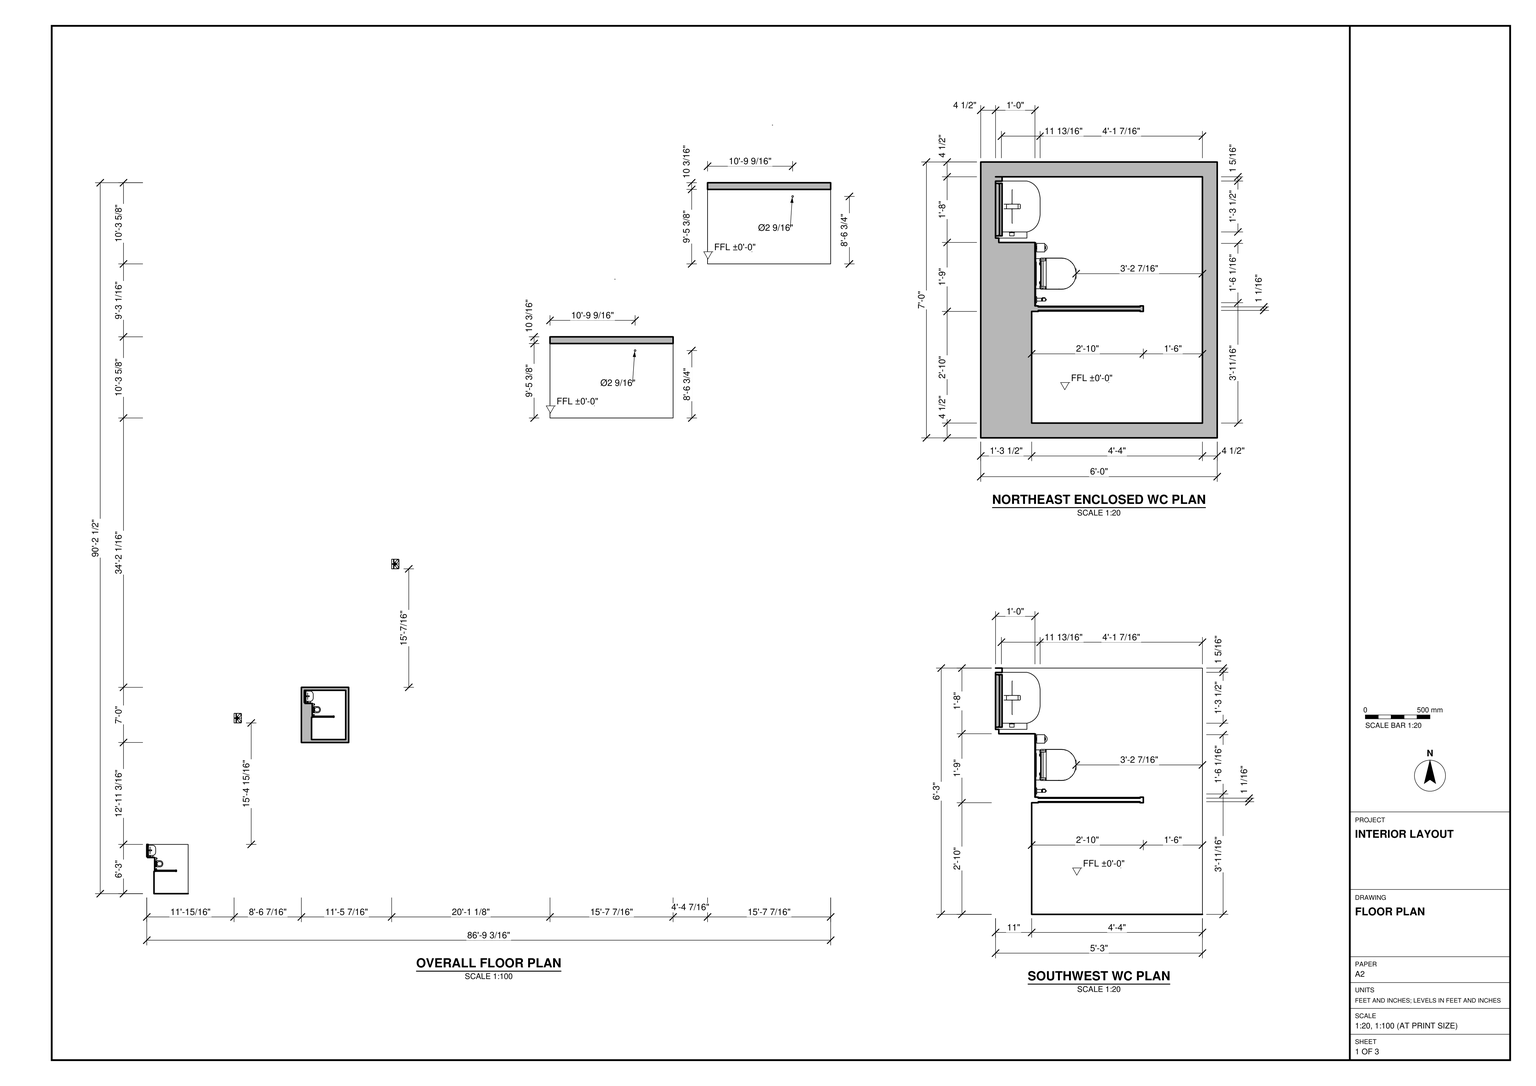
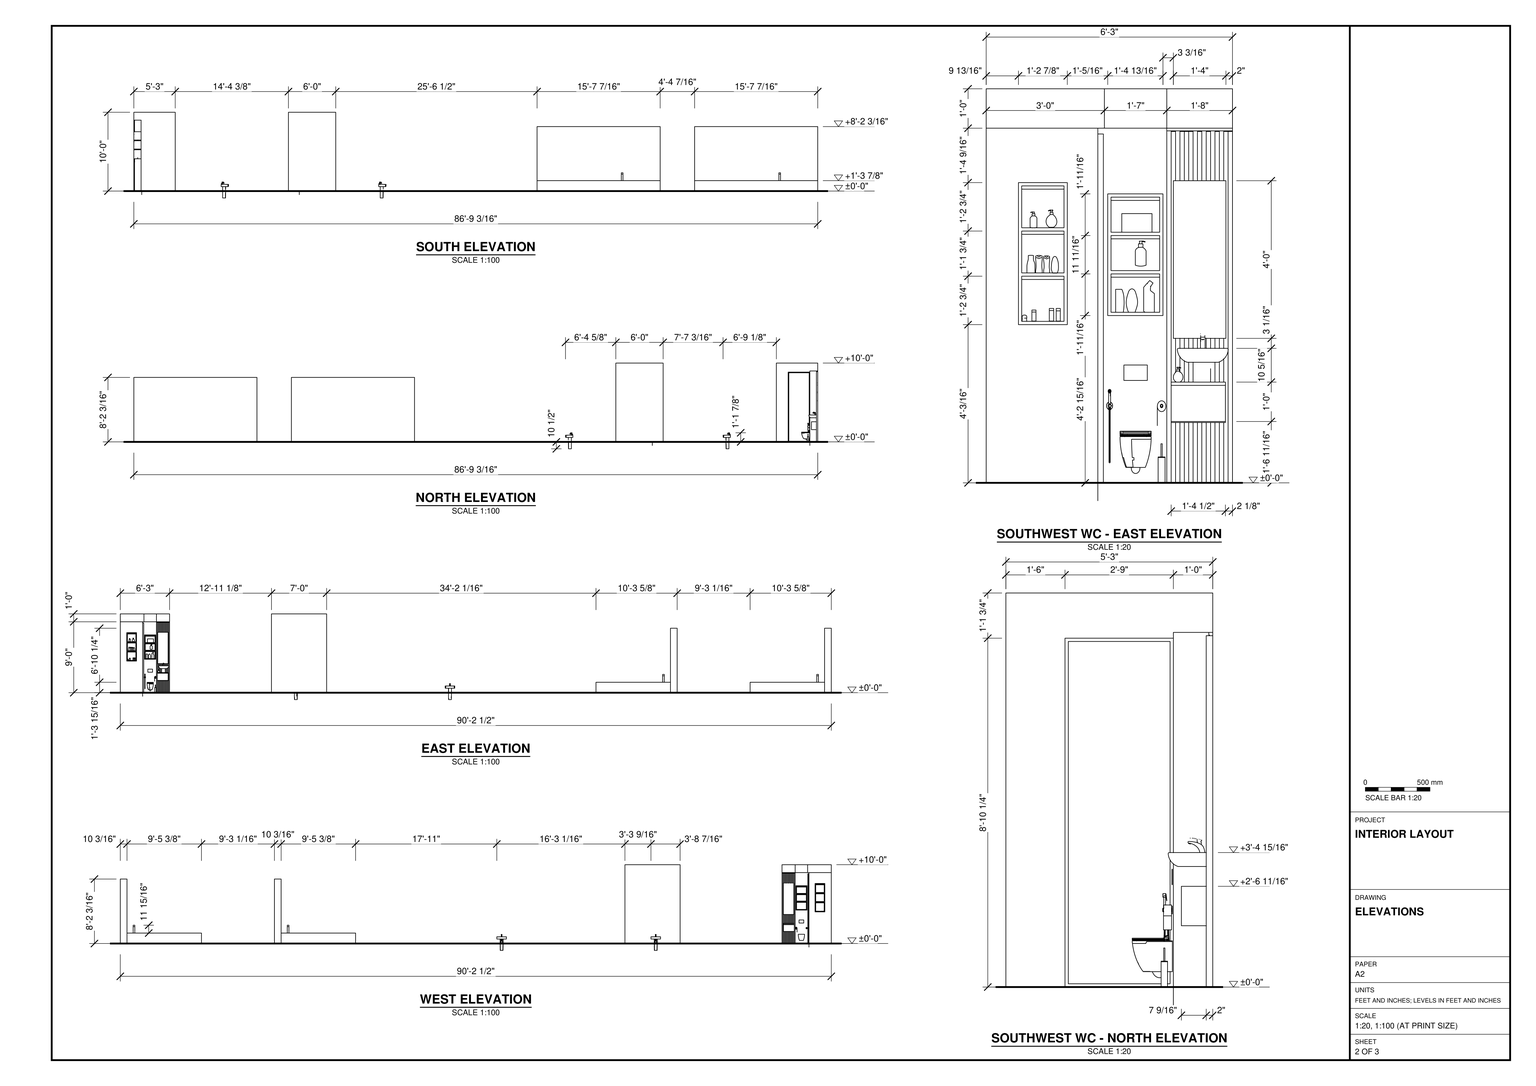
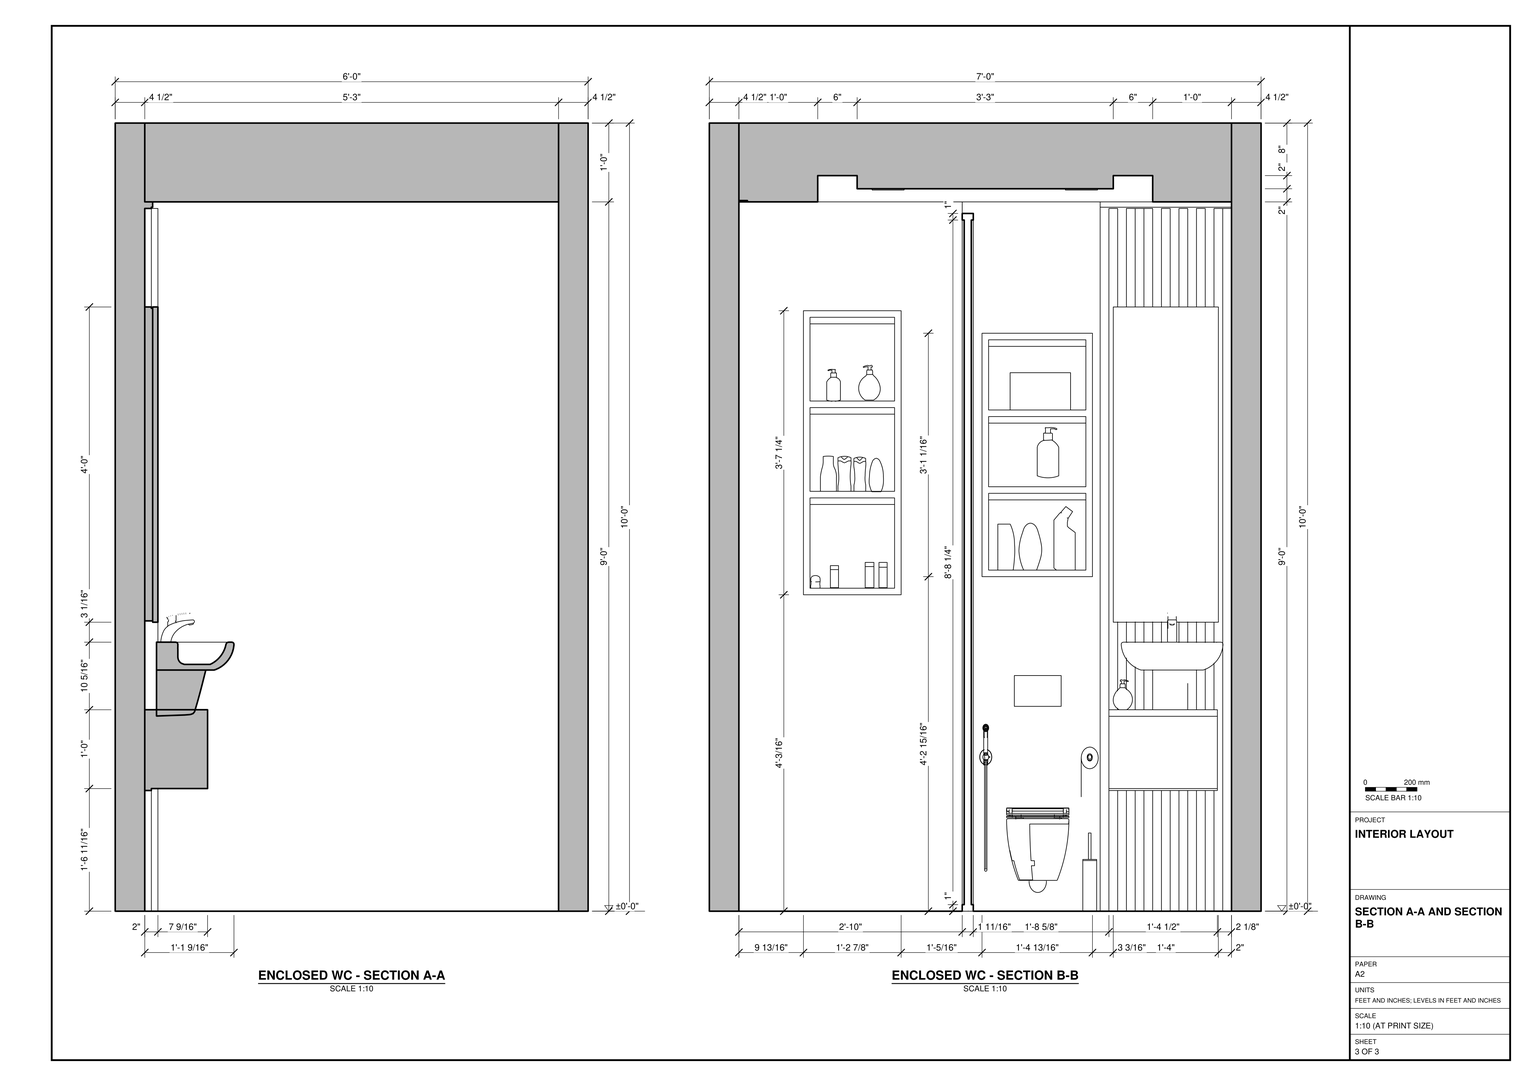
Build the interior layout in SketchUp from task_files/diagram_01.pdf. Work in feet and inches. Use the overall plan to position the separate assemblies; the spaces between them are part of the layout. The overall size is 86'-9 3/16" along x, 90'-2 1/2" along y and 10'-10 1/2" along z. Use the single finished floor level of ±0'-0".

Model the open southwest WC and the enclosed WC to its northeast. Use the enlarged plans for the stepped fixture wall and projecting partition. For the enclosed version, use the sections to set the perimeter wall thickness, ceiling height and stepped underside of the top slab. Fit both layouts with the wall-hung toilet, basin and tap, suspended cabinet, mirror, vertically lined backing and recessed shelves. Match the shelf sizes and the elevations of the basin fittings to the detail drawings. Decor and loose items, including containers on the shelves, may be any suitable library components.

Include the detached basin fixtures and the two larger rectangular assemblies farther northeast, each with a low base and a tall end panel. Keep the shell elements, including walls and slabs, and each furniture or joinery piece in separate groups or components. Use components for repeated parts. Save one SketchUp model as output_files/open_and_enclosed_wc_layouts_and_separate_fixtures.skp.

# SketchUp Ruby script. Lengths in inches.
U = 1.inch
M = Sketchup.active_model
def pt(a) = Geom::Point3d.new(a.map { |v| v * U })
def face(e, loops, mat)
  f = e.add_face(loops[0].map { |a| pt(a) })
  loops[1..].each { |l| e.add_face(l.map { |a| pt(a) }).erase! }
  f.material = f.back_material = mat if mat
  f
end
# faces: each face lists its corners as indices into pts; further lists are holes
def faces(e, pts, list, mat = nil) = list.each { |f| face(e, (f[0].is_a?(Array) ? f : [f]).map { |l| l.map { |i| pts[i] } }, mat) }
# xy, xz, yz: faces in a plane at the given z, y or x. An outline is a flat list of corners, or four numbers for a rectangle; further outlines are holes
def ring(l) = l.size == 4 ? [[l[0], l[1]], [l[2], l[1]], [l[2], l[3]], [l[0], l[3]]] : l.each_slice(2).to_a
def flat(e, list, mat, &to3) = list.each { |f| face(e, (f[0].is_a?(Array) ? f : [f]).map { |l| ring(l).map { |u, v| to3.(u, v) } }, mat) }
def xy(e, z, list, mat = nil) = flat(e, list, mat) { |x, y| [x, y, z] }
def xz(e, y, list, mat = nil) = flat(e, list, mat) { |x, z| [x, y, z] }
def yz(e, x, list, mat = nil) = flat(e, list, mat) { |y, z| [x, y, z] }
def lines(e, pts, list) = list.each { |a, b| e.add_line(pt(pts[a]), pt(pts[b])) }
# prism: a flat outline (further loops are holes) pulled along v
def prism(e, loops, v, mat = nil)
  f = face(e, loops, mat); d = Geom::Vector3d.new(v.map { |x| x * U })
  f.pushpull(f.normal.samedirection?(d) ? d.length : -d.length)
end
def box(e, o, s, mat = nil) = prism(e, [[o, [o[0] + s[0], o[1], o[2]], [o[0] + s[0], o[1] + s[1], o[2]], [o[0], o[1] + s[1], o[2]]]], [0, 0, s[2]], mat)
def at(x, y, z, deg = 0) = Geom::Transformation.translation(pt([x, y, z])) * Geom::Transformation.rotation(ORIGIN, Z_AXIS, deg.degrees)
def axes(o, x, y, z) = Geom::Transformation.new([*x, 0, *y, 0, *z, 0, *pt(o).to_a, 1])
def part(name) = M.definitions.add(name)
# library, detail: a bought-in or finely detailed component or shape, given as its bounding box
def library(name, o, s) = part(name).tap { |d| box(d.entities, o, s) }
def detail(e, o, s) = box(e.add_group.entities, o, s)
def put(e, d, t, mat = nil) = e.add_instance(d, t).tap { |i| i.material = mat if mat }
def group(e, t, mat = nil) = e.add_group.tap { |g| g.transformation = t; g.material = mat if mat }.entities
root = M.entities
M.materials.add("[0020_Red]").color = [255, 0, 0]
M.materials.add("[Carrera Marble]").color = [207, 207, 207]
M.materials.add("[Color M09]").color = [0, 0, 0]
M.materials.add("[Color_000]").color = [255, 234, 104]
M.materials.add("[Color_A02]").color = [255, 50, 50]
M.materials.add("[Color_B06]").color = [163, 8, 0]
M.materials.add("[Color_C10]").color = [125, 119, 117]
M.materials.add("[Color_I11]").color = [2, 32, 114]
M.materials.add("[Mirror 01]").color = [185, 185, 185]
M.materials.add("[Terrazzo Tile Accent]").color = [224, 221, 217]
M.materials.add("[Translucent Glass Sky Reflection]").color = [126, 138, 183]
M.materials["[Translucent Glass Sky Reflection]"].alpha = 0.52
M.materials.add("[Wood Veneer 01]").color = [120, 70, 37]
c1 = library("Wall-hung toilet assembly",[0,0,0],[28.35,19.69,42.125])
c2 = library("33.dxf",[36.1875,14.52,12],[23.625,39.43,18.1])
c3 = library("washbasin-1",[-10.81,-16.44,-15.75],[21.62,16.44,23.34])
c4 = library("Group\#4",[0,0,0],[5.59,14.85,1.64])
c5 = library("Group\#6",[0,0,0],[7.39,15.23,1.95])
c6 = library("Group\#10",[0,0,-0.06],[5.12,14.5,1.72])
c7 = library("Group\#7",[0,0,0],[9.4,15.15,3.11])
c8 = library("Group\#11",[0,0,0],[9.4,3.11,15.15])
c9 = library("Group\#12",[0,0,0],[5.95,13.93,3.02])
c10 = library("Group\#13",[0,0,0],[5.95,13.93,3.02])
c11 = library("Group\#16",[0,0,0],[6.09,14.19,2.01])
c12 = library("Group\#17",[0,0,0],[5.65,13.74,2.92])
c13 = part("Restroom layouts")
xy(c13.entities,0,[[613.9,724.22,627.35,837.63],[784.39,724.22,801.34,837.63],[613.9,837.63,627.35,847.82],[784.39,837.63,801.34,847.82]])
xy(c13.entities,0,[[11,0,63,0,63,75,2,75,2,73.67,0,73.67,0,72.33,1,72.33,1,71,0,71,0,69.67,1,69.67,1,68.33,0,68.33,0,67,1,67,1,65.67,0,65.67,0,64.33,1,64.33,1,63,0,63,0,61.67,1,61.67,1,60.33,0,60.33,0,59,1,59,1,57.67,0,57.67,0,56.33,1,56.33,1,55,12,55,12,35.68,45,35.68,45,34,11,34]],"[Terrazzo Tile Accent]")
xy(c13.entities,1,[[13,34,44,34.3],[13,35.38,44,35.68]],"[Color M09]")
xy(c13.entities,15.92,[[613.9,724.22,801.34,837.63]],"[Color_C10]")
xy(c13.entities,18.37,[[0,56.33,1,57.67],[0,57.67,1,59],[0,59,1,60.33],[0,60.33,1,61.67],[0,61.67,1,63],
  [0,63,1,64.33],[0,64.33,1,65.67],[0,65.67,1,67],[0,67,1,68.33],[0,68.33,1,69.67],
  [0,69.67,1,71],[0,71,1,72.33],[0,72.33,1,72.85]],"[Color_000]")
xy(c13.entities,18.67,[[1,56.33,9.5625,72.85]])
xy(c13.entities,30.67,[[0,56.33,9.5625,72.85]])
xy(c13.entities,44,[[1.2,57,2,73]])
xy(c13.entities,44.2,[[0,57,1,57.2],[0,72.8,1,73]])
xy(c13.entities,44.2,[[0,57.2,1.2,72.8]],"[Color_000]")
xy(c13.entities,49.18,[[0,10.83,11,23.7]])
xy(c13.entities,51.9375,[[0,38.02,12,52.83]])
xy(c13.entities,61.93,[[0,10.83,0.2,23.7]])
xy(c13.entities,62.625,[[0,38.02,0.2,52.83]])
xy(c13.entities,62.93,[[0.2,10.83,11,23.7]])
xy(c13.entities,63.625,[[0.2,38.02,12,52.83]])
xy(c13.entities,63.93,[[0,10.83,11,23.7]])
xy(c13.entities,64.625,[[0,38.02,12,52.83]])
xy(c13.entities,74.3125,[[0,38.02,0.2,52.83]])
xy(c13.entities,75.3125,[[0.2,38.02,12,52.83]])
xy(c13.entities,75.68,[[0,10.83,0.2,23.7]])
xy(c13.entities,76.3125,[[0,38.02,12,52.83]])
xy(c13.entities,76.68,[[0.2,10.83,11,23.7]])
xy(c13.entities,77.68,[[0,10.83,11,23.7]])
xy(c13.entities,86,[[0,38.02,0.2,52.83]])
xy(c13.entities,87,[[0.2,38.02,12,52.83]])
xy(c13.entities,89.43,[[0,10.83,0.2,23.7]])
xy(c13.entities,90.43,[[0.2,10.83,11,23.7]])
xy(c13.entities,91.8,[[1,57.2,1.2,72.8]],"[Color_000]")
xy(c13.entities,92,[[0,57,1,57.67],[1.2,57,2,73],[0,59,1,60.33],[0,61.67,1,63],[0,64.33,1,65.67],
  [0,67,1,68.33],[0,69.67,1,71],[0,72.33,1,73]])
xy(c13.entities,98.18,[[613.9,837.63,801.34,847.82]])
xy(c13.entities,105.24,[[13,34,44,34.3],[13,35.38,44,35.68]],"[Color M09]")
xy(c13.entities,106.24,[[12,34,45,35.68]],"[Color M09]")
xy(c13.entities,107,[[0,56.33,1,57.67],[0,59,1,60.33],[0,60.33,1,61.67],[0,61.67,1,63],[0,64.33,1,65.67],
  [0,67,1,68.33],[0,69.67,1,71],[0,72.33,1,73.67],[1,73.67,2,75]])
xy(c13.entities,107.1875,[[1,55,1.2,75]])
xy(c13.entities,108,[[0,0,11,0,11,34,12,34,12,55,0,55],[0,55,1.2,75]])
xz(c13.entities,0,[[11,0,11,108,0,108,0,120,63,120,63,0]],"[Carrera Marble]")
xz(c13.entities,10.83,[[0,49.18,0,61.93,0.2,61.93,0.2,62.93,11,62.93,11,49.18],[0,63.93,0,75.68,0.2,75.68,0.2,76.68,11,76.68,11,63.93],[0,77.68,0,89.43,0.2,89.43,0.2,90.43,11,90.43,11,77.68]])
xz(c13.entities,23.7,[[0,49.18,11,49.18,11,62.93,0.2,62.93,0.2,61.93,0,61.93],[0,63.93,11,63.93,11,76.68,0.2,76.68,0.2,75.68,0,75.68],[0,77.68,11,77.68,11,90.43,0.2,90.43,0.2,89.43,0,89.43]])
xz(c13.entities,34,[[11,0,12,108]])
xz(c13.entities,34,[[[12,0,45,106.24],[13,1,44,105.24]]],"[Color M09]")
xz(c13.entities,34.3,[[13,1,44,105.24]],"[Translucent Glass Sky Reflection]")
xz(c13.entities,35.38,[[13,1,44,105.24]],"[Translucent Glass Sky Reflection]")
xz(c13.entities,35.68,[[[12,0,45,106.24],[13,1,44,105.24]]],"[Color M09]")
xz(c13.entities,38.02,[[0,51.9375,0,62.625,0.2,62.625,0.2,63.625,12,63.625,12,51.9375],[0,64.625,0,74.3125,0.2,74.3125,0.2,75.3125,12,75.3125,12,64.625],[0,76.3125,0,86,0.2,86,0.2,87,12,87,12,76.3125]])
xz(c13.entities,52.83,[[0,51.9375,12,51.9375,12,63.625,0.2,63.625,0.2,62.625,0,62.625],[0,64.625,12,64.625,12,75.3125,0.2,75.3125,0.2,74.3125,0,74.3125],[0,76.3125,12,76.3125,12,87,0.2,87,0.2,86,0,86]])
xz(c13.entities,55,[[1,0,1,107.1875,1.2,107.1875,1.2,108,12,108,12,0]])
xz(c13.entities,56.33,[[0,0,1,18.37],[0,18.37,1,30.67],[1,18.67,9.5625,30.67],[0,30.67,1,107]])
xz(c13.entities,57,[[1.2,44,2,92],[0,44.2,1,92]])
xz(c13.entities,57.2,[[1,44.2,1.2,91.8]],"[Color_000]")
xz(c13.entities,57.67,[[0,0,1,18.37],[0,92,1,107]])
xz(c13.entities,59,[[0,0,1,18.37],[0,92,1,107]])
xz(c13.entities,60.33,[[0,0,1,18.37],[0,92,1,107]])
xz(c13.entities,61.67,[[0,0,1,18.37],[0,92,1,107]])
xz(c13.entities,63,[[0,0,1,18.37],[0,92,1,107]])
xz(c13.entities,64.33,[[0,0,1,18.37],[0,92,1,107]])
xz(c13.entities,65.67,[[0,0,1,18.37],[0,92,1,107]])
xz(c13.entities,67,[[0,0,1,18.37],[0,92,1,107]])
xz(c13.entities,68.33,[[0,0,1,18.37],[0,92,1,107]])
xz(c13.entities,69.67,[[0,0,1,18.37],[0,92,1,107]])
xz(c13.entities,71,[[0,0,1,18.37],[0,92,1,107]])
xz(c13.entities,72.33,[[0,0,1,18.37],[0,92,1,107]])
xz(c13.entities,72.8,[[1,44.2,1.2,91.8]],"[Color_000]")
xz(c13.entities,72.85,[[0,18.37,0,30.67,9.5625,30.67,9.5625,18.67,1,18.67,1,18.37]])
xz(c13.entities,73,[[1.2,44,2,92],[0,44.2,1,92]])
xz(c13.entities,73.67,[[0,0,2,107]])
xz(c13.entities,75,[[0,0,2,107],[0,107,0,108,1.2,108,1.2,107.1875,1,107.1875,1,107]])
xz(c13.entities,724.22,[[613.9,0,801.34,15.92]],"[Color_C10]")
xz(c13.entities,837.63,[[613.9,15.92,801.34,98.18]],"[Color_C10]")
xz(c13.entities,847.82,[[613.9,0,801.34,98.18]])
yz(c13.entities,0,[[56.33,0,57.67,18.37],[59,0,60.33,18.37],[61.67,0,63,18.37],[64.33,0,65.67,18.37],[67,0,68.33,18.37],
  [69.67,0,71,18.37],[72.33,0,73.67,0,73.67,107,72.33,107,72.33,92,73,92,73,44.2,72.33,44.2,72.33,30.67,72.85,30.67,72.85,18.37,72.33,18.37],[56.33,18.37,72.85,28.67],[56.33,28.67,57.67,30.67],[57.67,28.67,59,30.67],
  [59,28.67,60.33,30.67],[60.33,28.67,61.67,30.67],[61.67,28.67,63,30.67],[63,28.67,64.33,30.67],[64.33,28.67,65.67,30.67],
  [65.67,28.67,67,30.67],[67,28.67,68.33,30.67],[68.33,28.67,69.67,30.67],[69.67,28.67,71,30.67],[71,28.67,72.33,30.67],
  [72.33,28.67,72.85,30.67],[56.33,30.67,57.67,30.67,57.67,44.2,57,44.2,57,92,57.67,92,57.67,107,56.33,107],[59,30.67,60.33,44.2],[61.67,30.67,63,44.2],[64.33,30.67,65.67,44.2],
  [67,30.67,68.33,44.2],[69.67,30.67,71,44.2],[57,44.2,73,44.2,73,92,72.33,92,72.33,107,71,107,71,92,69.67,92,69.67,107,68.33,107,68.33,92,67,92,67,107,65.67,107,65.67,92,64.33,92,64.33,107,63,107,63,92,61.67,92,61.67,107,60.33,107,60.33,92,59,92,59,107,57.67,107,57.67,92,57,92],[10.83,49.18,23.7,61.93],[38.02,51.9375,52.83,62.625],
  [10.83,63.93,23.7,75.68],[38.02,64.625,52.83,74.3125],[38.02,76.3125,52.83,86],[10.83,77.68,23.7,89.43],[59,92,60.33,107],
  [61.67,92,63,107],[64.33,92,65.67,107],[67,92,68.33,107],[69.67,92,71,107],[0,108,36,120],
  [36,108,55,120],[55,108,75,120]])
yz(c13.entities,0,[[57.67,30.67,59,44.2],[60.33,30.67,61.67,44.2],[63,30.67,64.33,44.2],[65.67,30.67,67,44.2],[68.33,30.67,69.67,44.2],
  [71,30.67,72.33,44.2]],"[Wood Veneer 01]")
yz(c13.entities,0.2,[[10.83,61.93,23.7,62.93],[38.02,62.625,52.83,63.625],[38.02,74.3125,52.83,75.3125],[10.83,75.68,23.7,76.68],[38.02,86,52.83,87],
  [10.83,89.43,23.7,90.43]],"[Color_000]")
yz(c13.entities,1,[[56.33,18.37,72.85,18.67],[57,44.2,57.2,91.8],[72.8,44.2,73,92],[57,91.8,57.67,92],[59,91.8,60.33,92],
  [61.67,91.8,63,92],[64.33,91.8,65.67,92],[67,91.8,68.33,92],[69.67,91.8,71,92],[72.33,91.8,72.8,92]])
yz(c13.entities,1,[[55,0,56.33,0,56.33,107,57.67,107,57.67,91.8,59,91.8,59,107,63,107,63,91.8,64.33,91.8,64.33,107,65.67,107,65.67,91.8,67,91.8,67,107,68.33,107,68.33,91.8,69.67,91.8,69.67,107,71,107,71,91.8,72.33,91.8,72.33,107,75,107,75,107.1875,55,107.1875],[57.67,0,59,18.37],[60.33,0,61.67,18.37],[63,0,64.33,18.37],[65.67,0,67,18.37],
  [68.33,0,69.67,18.37],[71,0,72.33,18.37],[60.33,91.8,61.67,107]],"[Wood Veneer 01]")
yz(c13.entities,1.2,[[57,44,73,44.2],[57,44.2,57.2,91.8],[57.2,44.2,72.8,91.8],[72.8,44.2,73,92],[57,91.8,72.8,92]])
yz(c13.entities,1.2,[[55,107.1875,75,108]],"[Color_000]")
yz(c13.entities,2,[[57,44,73,92]],"[Mirror 01]")
yz(c13.entities,2,[[73.67,0,75,107]],"[Wood Veneer 01]")
yz(c13.entities,9.5625,[[56.33,18.67,72.85,29.67],[56.33,29.67,72.85,30.67]])
yz(c13.entities,11,[[[9.83,48.18,24.7,91.43],[10.83,49.18,23.7,62.93],[10.83,63.93,23.7,76.68],[10.83,77.68,23.7,90.43]]])
yz(c13.entities,11,[[[0,0,34,108],[9.83,48.18,24.7,91.43]]],"[Carrera Marble]")
yz(c13.entities,12,[[[37.02,50.9375,53.83,88],[38.02,51.9375,52.83,63.625],[38.02,76.3125,52.83,87],[38.02,64.625,52.83,75.3125]]])
yz(c13.entities,12,[[[35.68,0,55,0,55,108,34,108,34,106.24,35.68,106.24],[37.02,50.9375,53.83,88]]],"[Carrera Marble]")
yz(c13.entities,13,[[34,1,34.3,105.24],[35.38,1,35.68,105.24]],"[Color M09]")
yz(c13.entities,44,[[34,1,34.3,105.24],[35.38,1,35.68,105.24]],"[Color M09]")
yz(c13.entities,45,[[34,0,35.68,106.24]],"[Color M09]")
yz(c13.entities,613.9,[[724.22,0,837.63,15.92],[837.63,0,847.82,98.18]])
yz(c13.entities,801.34,[[724.22,0,837.63,15.92],[837.63,0,847.82,98.18]])
p = [[12,34,0],[12,34,-5.45],[712.46,935.57,0],[713.08,935.57,0]]
lines(c13.entities,p,[[0,1],[2,3]])
put(c13.entities,c1,axes([12.31,55,0],[0,-0.67028,0],[0.62169,0,0],[0,0,0.85172]))
put(c13.entities,c2,axes([125.49,237.5,-19.52],[0,0.62,0],[0,0,0.62],[0.62,0,0]))
put(c13.entities,c3,axes([1.79,65.96,40.96],[0,0.7168,0],[-0.7168,0,0],[0,0,0.7168]))
g1 = group(c13.entities,at(6.3125,41.29,76.3125))
xy(g1,0,[[0,0,1.99,9.2]])
xy(g1,5.68,[[0,0,1.99,9.2]])
xz(g1,0,[[0,0,1.99,2.09],[0,2.09,1.99,5.68]])
xz(g1,9.2,[[0,0,1.99,2.09],[0,2.09,1.99,5.68]])
yz(g1,0,[[0,0,9.2,5.68]])
yz(g1,1.99,[[0,0,9.2,2.09],[0,2.09,9.2,5.68]])
g2 = group(c13.entities,at(6.6,42,51.9375),"[Color_A02]")
xy(g2,0,[[-0.94,-2.58,0,-0.25]],"[Color_B06]")
xy(g2,7,[[-0.94,-2.58,0,-0.7]],"[Color_B06]")
xz(g2,-2.58,[[-0.94,0,0,7]],"[Color_B06]")
xz(g2,0,[[-0.94,2.64,0,3.09]],"[Color_B06]")
yz(g2,-0.94,[[-2.58,0,-2.58,7,-0.7,7,-0.59,6.76,-0.5,6.52,-0.41,6.27,-0.27,5.77,-0.21,5.52,-0.16,5.26,-0.12,5.01,-0.08,4.75,-0.06,4.49,-0.04,3.97,-0.01,3.53,0,3.09,0,2.64,-0.02,2.2,-0.06,1.76,-0.1,1.17,-0.17,0.58,-0.25,0]])
yz(g2,0,[[-2.58,0,-0.25,0,-0.17,0.58,-0.1,1.17,-0.06,1.76,-0.02,2.2,0,2.64,0,3.09,-0.01,3.53,-0.04,3.97,-0.06,4.49,-0.08,4.75,-0.12,5.01,-0.16,5.26,-0.21,5.52,-0.27,5.77,-0.41,6.27,-0.5,6.52,-0.59,6.76,-0.7,7,-2.58,7]])
p = [[0,-0.17,0.58],[0,-0.25,0],[-0.94,-0.25,0],[-0.94,-0.17,0.58],[0,-0.1,1.17],[-0.94,-0.1,1.17],
  [0,-0.06,1.76],[-0.94,-0.06,1.76],[0,-0.02,2.2],[-0.94,-0.02,2.2],[0,0,2.64],[-0.94,0,2.64],
  [0,-0.01,3.53],[0,0,3.09],[-0.94,0,3.09],[-0.94,-0.01,3.53],[0,-0.04,3.97],[-0.94,-0.04,3.97],
  [0,-0.05,4.23],[-0.94,-0.05,4.23],[0,-0.06,4.49],[-0.94,-0.06,4.49],[0,-0.08,4.75],[-0.94,-0.08,4.75],
  [0,-0.12,5.01],[-0.94,-0.12,5.01],[0,-0.16,5.26],[-0.94,-0.16,5.26],[0,-0.21,5.52],[-0.94,-0.21,5.52],
  [0,-0.27,5.77],[-0.94,-0.27,5.77],[0,-0.34,6.02],[-0.94,-0.34,6.02],[0,-0.41,6.27],[-0.94,-0.41,6.27],
  [0,-0.5,6.52],[-0.94,-0.5,6.52],[0,-0.59,6.76],[-0.94,-0.59,6.76],[0,-0.7,7],[-0.94,-0.7,7]]
faces(g2,p,[[0,1,2,3],[4,0,3,5],[6,4,5,7],[8,6,7,9],[10,8,9,11],[12,13,14,15],[16,12,15,17],[18,16,17,19],
  [20,18,19,21],[22,20,21,23],[24,22,23,25],[26,24,25,27],[28,26,27,29],[30,28,29,31],[32,30,31,33],[34,32,33,35],
  [36,34,35,37],[38,36,37,39],[40,38,39,41]],"[Color_B06]")
g3 = group(c13.entities,at(6.77,51.21,51.77))
xy(g3,0,[[-1.27,-2.66,0,-0.16]],"[Color_I11]")
xy(g3,8.89,[[-0.18,-2.26,0,-2.26,0,-2.07]],"[Color_I11]")
xz(g3,-3.25,[[-1.27,0.49,0,7.78]],"[Color_I11]")
xz(g3,-1.2,[[-1.27,6.85,0,6.99],[-1.27,6.99,0,7.43]],"[Color_I11]")
xz(g3,0,[[-1.27,0.17,0,5.88]],"[Color_I11]")
yz(g3,-1.27,[[-2.66,0,-3.25,0.49,-3.25,7.78,-3.01,8.06,-2.34,8.86,-2.26,8.89,-2.15,8.8125,-1.2,8.1,-1.09,8.03,-1.2,7.43,-1.2,6.85,-1.02,6.65,-0.12,5.97,0,5.88,0,0.17,-0.16,0]])
yz(g3,-1.27,[[-1.2,8.1,-2.15,8.8125,-1.3125,9.76,-0.49,9.14]],"[0020_Red]")
yz(g3,0,[[-2.66,0,-0.16,0,0,0.17,0,5.88,-0.12,5.97,-1.02,6.65,-1.2,6.85,-1.2,7.43,-1.09,8.03,-1.22,8.14,-2.07,8.89,-2.26,8.89,-2.34,8.86,-3.01,8.06,-3.25,7.78,-3.25,0.49]])
yz(g3,0,[[-1.22,8.14,-0.51,9.16,-1.3125,9.76,-2.07,8.89]],"[0020_Red]")
p = [[0,-2.66,0],[0,-3.25,0.49],[-1.27,-3.25,0.49],[-1.27,-2.66,0],[0,0,0.17],[0,-0.16,0],
  [-1.27,-0.16,0],[-1.27,0,0.17],[0,-0.12,5.97],[0,0,5.88],[-1.27,0,5.88],[-1.27,-0.12,5.97],
  [0,-1.02,6.65],[-1.27,-1.02,6.65],[0,-1.2,6.85],[-1.27,-1.2,6.85],[0,-1.09,8.03],[0,-1.2,7.43],
  [-1.27,-1.2,7.43],[-1.27,-1.09,8.03],[-1.16,-1.09,8.03],[-0.16,-1.09,8.03],[0,-3.25,7.78],[0,-3.01,8.06],
  [-1.27,-3.01,8.06],[-1.27,-3.25,7.78],[-1.27,-1.2,8.1],[-1.27,-0.49,9.14],[-0.17,-0.4,9.07],[0,-1.22,8.14],
  [-1.13,-0.4,9.07],[0,-2.34,8.86],[-1.27,-2.34,8.86],[0,-0.51,9.16],[-1.09,-1.43,9.84],[-1.27,-2.15,8.8125],
  [-1.16,-2.26,8.89],[-1.27,-2.26,8.89],[-1.27,-1.3125,9.76],[0,-2.26,8.89],[-0.18,-2.26,8.89],[-0.18,-1.43,9.84],
  [0,-2.07,8.89],[0,-1.3125,9.76],[-1.09,-2.28,8.88]]
faces(g3,p,[[0,1,2,3],[4,5,6,7],[8,9,10,11],[12,8,11,13],[14,12,13,15],[16,17,18,19,20,21],[22,23,24,25],[26,20,19],
  [21,29,16],[23,31,32,24],[36,35,37],[31,39,40,36,37,32]],"[Color_I11]")
faces(g3,p,[[27,20,26],[28,29,21],[20,27,30],[21,20,30,28],[29,28,33],[34,35,36],[35,34,38],[41,34,36,40],
  [40,42,43,41],[34,41,43,33,28,30,27,38]],"[0020_Red]")
lines(g3,p,[[44,27]])
put(c13.entities,c4,axes([6.26,15.07,63.93],[0,0.3596,0],[0,0,0.3596],[0.3596,0,0]))
g4 = group(c13.entities,at(6.78,14.86,63.93))
detail(g4,[-1.08,-2.45,0],[1.08,2.45,5.36])
put(c13.entities,c5,axes([6.55,46.1,51.92],[0,-0.47,0],[0,0,0.47],[-0.47,0,0]))
g5 = group(c13.entities,at(3.54,20.51,49.26))
detail(g5,[0.07,-1.28,0],[1.84,1.33,3.85])
g6 = group(c13.entities,at(3.25,21.45,49.26))
detail(g6,[0.16,-0.125,0],[1.72,1.25,3.85])
put(c13.entities,c6,axes([6.73,19.33,63.93],[0,-0.3596,0],[0,0,0.3596],[-0.3596,0,0]))
put(c13.entities,c7,axes([4.23,56.99,30.67],[0,0.31149,0],[0,0,0.30175],[0.4867,0,0]))
put(c13.entities,c8,axes([6.3,18.23,77.82],[0,0.35,0],[-0.35,0,0],[0,0,0.35]))
put(c13.entities,c9,axes([12,48.7,65.99],[0,-0.55,0],[0,0,0.55],[-0.55,0,0]))
put(c13.entities,c10,axes([4.82,13.37,77.63],[0,0.35,0],[0,0,0.35],[0.35,0,0]))
g7 = group(c13.entities,at(743.45,825.19,15.92,45))
detail(g7,[0,0,0],[2.54,2.54,11.95])
g8 = group(c13.entities,at(5.03,15.38,49.26))
detail(g8,[-0.46,-1.46,0],[1.72,1.25,3.36])
put(c13.entities,c11,axes([6.78,22.01,63.87],[0,-0.3596,0],[0,0,0.3596],[-0.3596,0,0]))
put(c13.entities,c12,axes([5,10.93,49.18],[-0.02405,0.24599,0],[0,0,0.14042],[0.34165,0.01731,0]))
c14 = library("Group\#18",[0,0,0],[63,75,12])
xy(root,0,[[235.375,230.16,235.375,314.16,307.375,314.16,307.375,300.31,302.875,300.31,302.875,309.66,239.875,309.66,239.875,234.66,302.875,234.66,302.875,266.39,307.375,266.39,307.375,230.16],[302.875,266.39,307.375,300.31]])
xy(root,108,[[250.875,234.66,302.875,235.95]])
xy(root,108.2,[[250.875,234.66,302.875,235.95]])
xy(root,120,[[[235.375,230.16,307.375,314.16],[239.875,234.66,302.875,309.66]]])
xz(root,230.16,[[235.375,0,307.375,120]])
xz(root,234.66,[[250.875,108,302.875,108.2]])
xz(root,235.95,[[250.875,108,302.875,108.2]])
xz(root,309.66,[[239.875,0,302.875,120]],"[Carrera Marble]")
xz(root,314.16,[[235.375,0,307.375,120]])
yz(root,235.375,[[230.16,0,314.16,120]])
yz(root,250.875,[[234.66,108,235.95,108.2]])
yz(root,302.875,[[234.66,0,234.66,108,235.95,108,235.95,108.2,234.66,108.2,234.66,120,309.66,120,309.66,0],[234.66,108,235.95,108.2]])
yz(root,307.375,[[230.16,0,314.16,120]])
put(root,c13,at(239.875,234.66,0))
put(root,c13,at(0,0,0))
put(root,c14,axes([239.875,234.66,120],[1,0,0],[0,1,0],[0,0,-1]))
